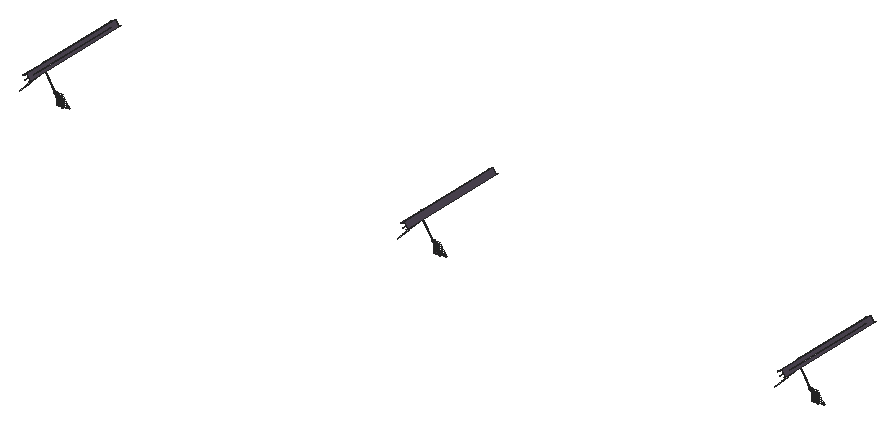
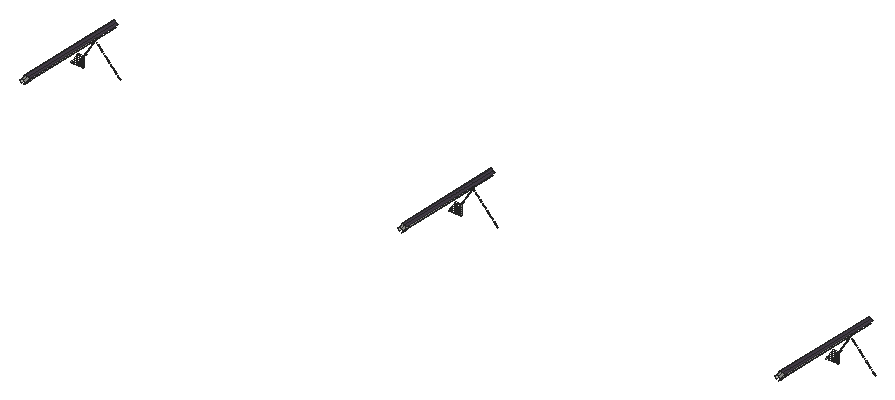
# SketchUp Ruby script. Lengths in inches.
U = 1.inch
M = Sketchup.active_model
def pt(a) = Geom::Point3d.new(a.map { |v| v * U })
def face(e, loops, mat)
  f = e.add_face(loops[0].map { |a| pt(a) })
  loops[1..].each { |l| e.add_face(l.map { |a| pt(a) }).erase! }
  f.material = f.back_material = mat if mat
  f
end
# faces: each face lists its corners as indices into pts; further lists are holes
def faces(e, pts, list, mat = nil) = list.each { |f| face(e, (f[0].is_a?(Array) ? f : [f]).map { |l| l.map { |i| pts[i] } }, mat) }
# xy, xz, yz: faces in a plane at the given z, y or x. An outline is a flat list of corners, or four numbers for a rectangle; further outlines are holes
def ring(l) = l.size == 4 ? [[l[0], l[1]], [l[2], l[1]], [l[2], l[3]], [l[0], l[3]]] : l.each_slice(2).to_a
def flat(e, list, mat, &to3) = list.each { |f| face(e, (f[0].is_a?(Array) ? f : [f]).map { |l| ring(l).map { |u, v| to3.(u, v) } }, mat) }
def xy(e, z, list, mat = nil) = flat(e, list, mat) { |x, y| [x, y, z] }
def xz(e, y, list, mat = nil) = flat(e, list, mat) { |x, z| [x, y, z] }
def yz(e, x, list, mat = nil) = flat(e, list, mat) { |y, z| [x, y, z] }
def lines(e, pts, list) = list.each { |a, b| e.add_line(pt(pts[a]), pt(pts[b])) }
# prism: a flat outline (further loops are holes) pulled along v
def prism(e, loops, v, mat = nil)
  f = face(e, loops, mat); d = Geom::Vector3d.new(v.map { |x| x * U })
  f.pushpull(f.normal.samedirection?(d) ? d.length : -d.length)
end
def box(e, o, s, mat = nil) = prism(e, [[o, [o[0] + s[0], o[1], o[2]], [o[0] + s[0], o[1] + s[1], o[2]], [o[0], o[1] + s[1], o[2]]]], [0, 0, s[2]], mat)
def at(x, y, z, deg = 0) = Geom::Transformation.translation(pt([x, y, z])) * Geom::Transformation.rotation(ORIGIN, Z_AXIS, deg.degrees)
def axes(o, x, y, z) = Geom::Transformation.new([*x, 0, *y, 0, *z, 0, *pt(o).to_a, 1])
def part(name) = M.definitions.add(name)
# library, detail: a bought-in or finely detailed component or shape, given as its bounding box
def library(name, o, s) = part(name).tap { |d| box(d.entities, o, s) }
def detail(e, o, s) = box(e.add_group.entities, o, s)
def put(e, d, t, mat = nil) = e.add_instance(d, t).tap { |i| i.material = mat if mat }
def group(e, t, mat = nil) = e.add_group.tap { |g| g.transformation = t; g.material = mat if mat }.entities
root = M.entities
M.materials.add("[Color M06]").color = [79, 71, 84]
xy(root,386.37,[[578.05,524.25,594.63,526.125],[1464.52,524.25,1481.09,526.125],[2350.98,524.25,2367.56,526.125]])
xy(root,387.5,[[578.05,524.25,593.91,526.125],[1464.52,524.25,1480.37,526.125],[2350.98,524.25,2366.84,526.125]])
xy(root,390.62,[[578.05,524.25,591.9,526.125],[1464.52,524.25,1478.37,526.125],[2350.98,524.25,2364.83,526.125]])
xy(root,391.75,[[578.05,524.25,591.18,526.125],[1464.52,524.25,1477.65,526.125],[2350.98,524.25,2364.11,526.125]])
xy(root,394.87,[[578.05,524.25,589.18,526.125],[1464.52,524.25,1475.64,526.125],[2350.98,524.25,2362.11,526.125]])
xy(root,396,[[578.05,524.25,588.46,526.125],[1464.52,524.25,1474.92,526.125],[2350.98,524.25,2361.39,526.125]])
xy(root,399.12,[[578.05,524.25,586.45,526.125],[1464.52,524.25,1472.92,526.125],[2350.98,524.25,2359.38,526.125]])
xy(root,400.25,[[578.05,524.25,585.73,526.125],[1464.52,524.25,1472.2,526.125],[2350.98,524.25,2358.66,526.125]])
xy(root,403.37,[[578.05,524.25,583.73,526.125],[1464.52,524.25,1470.19,526.125],[2350.98,524.25,2356.66,526.125]])
xy(root,404.5,[[578.05,524.25,583.01,526.125],[1464.52,524.25,1469.47,526.125],[2350.98,524.25,2355.9375,526.125]])
xy(root,407.62,[[578.05,524.25,581,526.125],[1464.52,524.25,1467.47,526.125],[2350.98,524.25,2353.93,526.125]])
xy(root,412.22,[[576.3,519.6875,578.05,521.5625],[1462.77,519.6875,1464.52,521.5625],[2349.23,519.6875,2350.98,521.5625],[576.3,521.5625,578.05,526.125],[1462.77,521.5625,1464.52,526.125],
  [2349.23,521.5625,2350.98,526.125]])
xz(root,521.5625,[[594.22,386.19,592.58,388.75,592.95,388.98,594.59,386.43],[1480.6875,386.19,1479.05,388.75,1479.42,388.98,1481.05,386.43],[2367.15,386.19,2365.51,388.75,2365.88,388.98,2367.52,386.43],[494.94,387.25,497.36,389.82,496.9,390.25,494.48,387.68],[1381.4,387.25,1383.82,389.82,1383.37,390.25,1380.94,387.68],
  [2267.86,387.25,2270.28,389.82,2269.83,390.25,2267.41,387.68],[592.03,389.61,590.39,392.17,590.76,392.4,592.4,389.85],[1478.49,389.61,1476.86,392.17,1477.22,392.4,1478.86,389.85],[2364.96,389.61,2363.32,392.17,2363.6875,392.4,2365.33,389.85],[498.23,390.75,500.66,393.33,500.2,393.75,497.78,391.18],
  [1384.7,390.75,1387.12,393.33,1386.66,393.75,1384.24,391.18],[2271.16,390.75,2273.58,393.33,2273.13,393.75,2270.71,391.18],[589.84,393.03,588.2,395.59,588.57,395.82,590.21,393.27],[1476.3,393.03,1474.66,395.59,1475.03,395.82,1476.67,393.27],[2362.77,393.03,2361.13,395.59,2361.5,395.82,2363.13,393.27],
  [501.53,394.26,503.95,396.83,503.5,397.26,501.08,394.6875],[1388,394.26,1390.42,396.83,1389.96,397.26,1387.54,394.6875],[2274.46,394.26,2276.88,396.83,2276.43,397.26,2274.01,394.6875],[587.64,396.45,586.01,399.01,586.375,399.24,588.01,396.69],[1474.11,396.45,1472.47,399.01,1472.84,399.24,1474.48,396.69],
  [2360.57,396.45,2358.94,399.01,2359.3,399.24,2360.94,396.69],[504.83,397.76,507.25,400.34,506.8,400.76,504.375,398.19],[1391.3,397.76,1393.72,400.34,1393.26,400.76,1390.84,398.19],[2277.76,397.76,2280.18,400.34,2279.73,400.76,2277.3,398.19],[585.45,399.875,583.81,402.43,584.18,402.66,585.82,400.11],
  [1471.92,399.875,1470.28,402.43,1470.65,402.66,1472.28,400.11],[2358.38,399.875,2356.74,402.43,2357.11,402.66,2358.75,400.11],[508.13,401.27,510.55,403.84,510.1,404.27,507.67,401.7],[1394.59,401.27,1397.01,403.84,1396.56,404.27,1394.14,401.7],[2281.06,401.27,2283.48,403.84,2283.02,404.27,2280.6,401.7],
  [583.26,403.29,581.62,405.85,581.99,406.08,583.63,403.53],[1469.72,403.29,1468.09,405.85,1468.45,406.08,1470.09,403.53],[2356.1875,403.29,2354.55,405.85,2354.92,406.08,2356.56,403.53],[511.43,404.77,513.85,407.34,513.39,407.77,510.97,405.2],[1397.89,404.77,1400.3125,407.34,1399.86,407.77,1397.4375,405.2],
  [2284.36,404.77,2286.78,407.34,2286.32,407.77,2283.9,405.2],[581.07,406.71,579.43,409.27,579.8,409.5,581.44,406.95],[1467.53,406.71,1465.89,409.27,1466.26,409.5,1467.9,406.95],[2354,406.71,2352.36,409.27,2352.73,409.5,2354.36,406.95],[514.73,408.28,517.15,410.85,516.69,411.28,514.27,408.7],
  [1401.19,408.28,1403.61,410.85,1403.16,411.28,1400.74,408.7],[2287.65,408.28,2290.08,410.85,2289.62,411.28,2287.2,408.7],[578.875,410.13,577.6875,411.99,578.05,412.22,579.24,410.37],[1465.34,410.13,1464.15,411.99,1464.52,412.22,1465.71,410.37],[2351.8,410.13,2350.61,411.99,2350.98,412.22,2352.17,410.37],
  [518.03,411.78,520.45,414.35,519.99,414.78,517.57,412.21],[1404.49,411.78,1406.91,414.35,1406.46,414.78,1404.03,412.21],[2290.95,411.78,2293.375,414.35,2292.92,414.78,2290.5,412.21],[577.6875,411.99,577.54,412.22,578.05,412.22],[1464.15,411.99,1464,412.22,1464.52,412.22],
  [2350.61,411.99,2350.46,412.22,2350.98,412.22],[577.54,412.22,578.05,412.22,577.61,412.92,577.24,412.6875],[1464,412.22,1464.52,412.22,1464.07,412.92,1463.7,412.6875],[2350.46,412.22,2350.98,412.22,2350.53,412.92,2350.16,412.6875],[576.68,413.55,577.05,413.79,575.86,415.64,575.49,415.41],
  [1463.15,413.55,1463.51,413.79,1462.33,415.64,1461.96,415.41],[2349.61,413.55,2349.98,413.79,2348.79,415.64,2348.42,415.41],[521.32,415.28,523.74,417.86,523.29,418.28,520.87,415.71],[1407.79,415.28,1410.21,417.86,1409.75,418.28,1407.33,415.71],[2294.25,415.28,2296.67,417.86,2296.22,418.28,2293.8,415.71],
  [575.49,415.41,575.86,415.64,575.41,416.34,575.04,416.11],[1461.96,415.41,1462.33,415.64,1461.875,416.34,1461.51,416.11],[2348.42,415.41,2348.79,415.64,2348.34,416.34,2347.97,416.11],[574.49,416.97,574.86,417.21,573.67,419.0625,573.3,418.83],[1460.95,416.97,1461.32,417.21,1460.13,419.0625,1459.77,418.83],
  [2347.42,416.97,2347.79,417.21,2346.6,419.0625,2346.23,418.83],[524.62,418.79,527.04,421.36,526.59,421.79,524.17,419.22],[1411.09,418.79,1413.51,421.36,1413.05,421.79,1410.63,419.22],[2297.55,418.79,2299.97,421.36,2299.52,421.79,2297.1,419.22],[573.3,418.83,573.67,419.0625,573.22,419.76,572.85,419.53],
  [1459.77,418.83,1460.13,419.0625,1459.68,419.76,1459.32,419.53],[2346.23,418.83,2346.6,419.0625,2346.15,419.76,2345.78,419.53],[572.3,420.39,572.66,420.63,571.48,422.48,571.11,422.25],[1458.76,420.39,1459.13,420.63,1457.94,422.48,1457.57,422.25],[2345.22,420.39,2345.59,420.63,2344.41,422.48,2344.04,422.25],
  [571.11,422.25,571.48,422.48,571.03,423.18,570.66,422.95],[1457.57,422.25,1457.94,422.48,1457.49,423.18,1457.12,422.95],[2344.04,422.25,2344.41,422.48,2343.96,423.18,2343.59,422.95],[527.92,422.29,530.34,424.86,529.89,425.29,527.47,422.72],[1414.38,422.29,1416.81,424.86,1416.35,425.29,1413.93,422.72],
  [2300.85,422.29,2303.27,424.86,2302.81,425.29,2300.39,422.72],[570.1,423.8125,570.47,424.05,569.28,425.9,568.92,425.67],[1456.57,423.8125,1456.9375,424.05,1455.75,425.9,1455.38,425.67],[2343.03,423.8125,2343.4,424.05,2342.21,425.9,2341.84,425.67],[568.92,425.67,569.28,425.9,568.83,426.6,568.47,426.37],
  [1455.38,425.67,1455.75,425.9,1455.3,426.6,1454.93,426.37],[2341.84,425.67,2342.21,425.9,2341.76,426.6,2341.39,426.37],[531.22,425.8,533.64,428.37,533.19,428.8,530.76,426.23],[1417.68,425.8,1420.1,428.37,1419.65,428.8,1417.23,426.23],[2304.15,425.8,2306.57,428.37,2306.11,428.8,2303.69,426.23],
  [567.91,427.23,568.28,427.47,567.09,429.32,566.72,429.09],[1454.375,427.23,1454.74,427.47,1453.56,429.32,1453.1875,429.09],[2340.84,427.23,2341.21,427.47,2340.02,429.32,2339.65,429.09],[566.72,429.09,567.09,429.32,566.64,430.02,566.27,429.79],[1453.1875,429.09,1453.56,429.32,1453.11,430.02,1452.74,429.79],
  [2339.65,429.09,2340.02,429.32,2339.57,430.02,2339.2,429.79],[534.52,429.3,536.9375,431.875,536.48,432.3,534.0625,429.73],[1420.98,429.3,1423.4,431.875,1422.95,432.3,1420.53,429.73],[2307.45,429.3,2309.87,431.875,2309.41,432.3,2306.99,429.73],[565.72,430.65,566.09,430.89,564.9,432.74,564.53,432.51],
  [1452.18,430.65,1452.55,430.89,1451.36,432.74,1451,432.51],[2338.65,430.65,2339.02,430.89,2337.83,432.74,2337.46,432.51],[564.53,432.51,564.9,432.74,564.45,433.44,564.08,433.21],[1451,432.51,1451.36,432.74,1450.91,433.44,1450.55,433.21],[2337.46,432.51,2337.83,432.74,2337.38,433.44,2337.01,433.21],
  [537.82,432.81,540.24,435.38,539.78,435.81,537.36,433.23],[1424.28,432.81,1426.7,435.38,1426.25,435.81,1423.83,433.23],[2310.74,432.81,2313.17,435.38,2312.71,435.81,2310.29,433.23],[563.53,434.07,563.89,434.31,562.71,436.16,562.34,435.93],[1449.99,434.07,1450.36,434.31,1449.17,436.16,1448.8,435.93],
  [2336.45,434.07,2336.82,434.31,2335.63,436.16,2335.27,435.93],[562.34,435.93,562.71,436.16,562.26,436.86,561.89,436.63],[1448.8,435.93,1449.17,436.16,1448.72,436.86,1448.35,436.63],[2335.27,435.93,2335.63,436.16,2335.18,436.86,2334.82,436.63],[541.12,436.31,543.54,438.88,543.08,439.31,540.66,436.74],
  [1427.58,436.31,1430,438.88,1429.55,439.31,1427.125,436.74],[2314.04,436.31,2316.46,438.88,2316.01,439.31,2313.59,436.74],[561.33,437.49,561.7,437.73,560.51,439.58,560.15,439.35],[1447.8,437.49,1448.17,437.73,1446.98,439.58,1446.61,439.35],[2334.26,437.49,2334.63,437.73,2333.44,439.58,2333.07,439.35],
  [560.15,439.35,560.51,439.58,560.0625,440.28,559.7,440.05],[1446.61,439.35,1446.98,439.58,1446.53,440.28,1446.16,440.05],[2333.07,439.35,2333.44,439.58,2332.99,440.28,2332.625,440.05],[544.41,439.8125,546.83,442.39,546.38,442.8125,543.96,440.24],[1430.88,439.8125,1433.3,442.39,1432.84,442.8125,1430.42,440.24],
  [2317.34,439.8125,2319.76,442.39,2319.31,442.8125,2316.89,440.24],[559.14,440.91,559.51,441.15,558.32,443,557.95,442.77],[1445.61,440.91,1445.97,441.15,1444.79,443,1444.42,442.77],[2332.07,440.91,2332.4375,441.15,2331.25,443,2330.88,442.77],[557.95,442.77,558.32,443,557.87,443.7,557.5,443.47],
  [1444.42,442.77,1444.79,443,1444.34,443.7,1443.97,443.47],[2330.88,442.77,2331.25,443,2330.8,443.7,2330.43,443.47],[547.71,443.32,550.13,445.89,549.68,446.32,547.26,443.75],[1434.18,443.32,1436.6,445.89,1436.14,446.32,1433.72,443.75],[2320.64,443.32,2323.0625,445.89,2322.61,446.32,2320.19,443.75],
  [556.95,444.33,557.32,444.57,556.13,446.42,555.76,446.1875],[1443.41,444.33,1443.78,444.57,1442.59,446.42,1442.22,446.1875],[2329.875,444.33,2330.24,444.57,2329.06,446.42,2328.6875,446.1875],[555.76,446.1875,556.13,446.42,555.68,447.125,555.3125,446.89],[1442.22,446.1875,1442.59,446.42,1442.14,447.125,1441.77,446.89],
  [2328.6875,446.1875,2329.06,446.42,2328.61,447.125,2328.24,446.89],[551.01,446.82,553.43,449.39,552.98,449.82,550.56,447.25],[1437.47,446.82,1439.9,449.39,1439.44,449.82,1437.02,447.25],[2323.9375,446.82,2326.36,449.39,2325.9,449.82,2323.48,447.25],[554.76,447.75,555.125,447.99,553.9375,449.84,553.57,449.61],
  [1441.22,447.75,1441.59,447.99,1440.4,449.84,1440.03,449.61],[2327.68,447.75,2328.05,447.99,2326.86,449.84,2326.5,449.61],[553.57,449.61,553.9375,449.84,553.56,450.4375,553.25,450.11],[1440.03,449.61,1440.4,449.84,1440.02,450.4375,1439.71,450.11],[2326.5,449.61,2326.86,449.84,2326.48,450.4375,2326.17,450.11],
  [553.25,450.11,553.1875,450.2,553.56,450.4375],[1439.71,450.11,1439.65,450.2,1440.02,450.4375],[2326.17,450.11,2326.11,450.2,2326.48,450.4375]])
xz(root,524.25,[[578.05,387.5,593.91,387.5,591.9,390.62,578.05,390.62],[1464.52,387.5,1480.37,387.5,1478.37,390.62,1464.52,390.62],[2350.98,387.5,2366.84,387.5,2364.83,390.62,2350.98,390.62],[578.05,391.75,591.18,391.75,589.18,394.87,578.05,394.87],[1464.52,391.75,1477.65,391.75,1475.64,394.87,1464.52,394.87],
  [2350.98,391.75,2364.11,391.75,2362.11,394.87,2350.98,394.87],[578.05,396,588.46,396,586.45,399.12,578.05,399.12],[1464.52,396,1474.92,396,1472.92,399.12,1464.52,399.12],[2350.98,396,2361.39,396,2359.38,399.12,2350.98,399.12],[578.05,400.25,585.73,400.25,583.73,403.37,578.05,403.37],
  [1464.52,400.25,1472.2,400.25,1470.19,403.37,1464.52,403.37],[2350.98,400.25,2358.66,400.25,2356.66,403.37,2350.98,403.37],[578.05,404.5,583.01,404.5,581,407.62,578.05,407.62],[1464.52,404.5,1469.47,404.5,1467.47,407.62,1464.52,407.62],[2350.98,404.5,2355.9375,404.5,2353.93,407.62,2350.98,407.62]],"[Color M06]")
xz(root,526.125,[[578.05,386.37,594.63,386.37,593.91,387.5,578.05,387.5],[1464.52,386.37,1481.09,386.37,1480.37,387.5,1464.52,387.5],[2350.98,386.37,2367.56,386.37,2366.84,387.5,2350.98,387.5],[604.81,387.5,607.53,387.5,605.53,390.62,602.8,390.62],[1491.27,387.5,1494,387.5,1491.99,390.62,1489.27,390.62],
  [2377.73,387.5,2380.46,387.5,2378.45,390.62,2375.73,390.62],[578.05,390.62,591.9,390.62,591.18,391.75,578.05,391.75],[1464.52,390.62,1478.37,390.62,1477.65,391.75,1464.52,391.75],[2350.98,390.62,2364.83,390.62,2364.11,391.75,2350.98,391.75],[578.05,394.87,589.18,394.87,588.46,396,578.05,396],
  [1464.52,394.87,1475.64,394.87,1474.92,396,1464.52,396],[2350.98,394.87,2362.11,394.87,2361.39,396,2350.98,396],[578.05,399.12,586.45,399.12,585.73,400.25,578.05,400.25],[1464.52,399.12,1472.92,399.12,1472.2,400.25,1464.52,400.25],[2350.98,399.12,2359.38,399.12,2358.66,400.25,2350.98,400.25],
  [578.05,403.37,583.73,403.37,583.01,404.5,578.05,404.5],[1464.52,403.37,1470.19,403.37,1469.47,404.5,1464.52,404.5],[2350.98,403.37,2356.66,403.37,2355.9375,404.5,2350.98,404.5],[578.05,407.62,581,407.62,580.125,409,578.05,409],[1464.52,407.62,1467.47,407.62,1466.59,409,1464.52,409],
  [2350.98,407.62,2353.93,407.62,2353.05,409,2350.98,409],[578.05,412.12,578.12,412.12,578.05,412.22],[1464.52,412.12,1464.58,412.12,1464.52,412.22],[2350.98,412.12,2351.05,412.12,2350.98,412.22]])
xz(root,526.125,[[578.05,409,580.125,409,578.12,412.12,578.05,412.12],[1464.52,409,1466.59,409,1464.58,412.12,1464.52,412.12],[2350.98,409,2353.05,409,2351.05,412.12,2350.98,412.12]],"[Color M06]")
xz(root,528.48,[[550.41,453.39,542.88,460.49,543.65,461.31,547.92,457.29],[550.41,453.39,547.92,457.29,551.1875,454.21],[1436.88,453.39,1429.34,460.49,1430.11,461.31,1434.38,457.29],[1436.88,453.39,1434.38,457.29,1437.65,454.21],[2323.34,453.39,2315.81,460.49,2316.58,461.31,2320.84,457.29],
  [2323.34,453.39,2320.84,457.29,2324.11,454.21],[551.1875,454.21,547.92,457.29,549.24,458.7,552.51,455.625],[1437.65,454.21,1434.38,457.29,1435.71,458.7,1438.98,455.625],[2324.11,454.21,2320.84,457.29,2322.17,458.7,2325.44,455.625],[547.92,457.29,543.65,461.31,544.98,462.72,549.24,458.7],
  [1434.38,457.29,1430.11,461.31,1431.44,462.72,1435.71,458.7],[2320.84,457.29,2316.58,461.31,2317.9,462.72,2322.17,458.7]])
xz(root,719.59,[[550.36,453.34,550.41,453.39,550.35,453.35],[1436.82,453.34,1436.88,453.39,1436.8125,453.35],[2323.29,453.34,2323.34,453.39,2323.28,453.35]])
xz(root,726.125,[[552.61,449.83,550.36,453.34,550.41,453.39,553.56,450.4375],[1439.07,449.83,1436.82,453.34,1436.88,453.39,1440.02,450.4375],[2325.54,449.83,2323.29,453.34,2323.34,453.39,2326.48,450.4375],[553.56,450.4375,550.41,453.39,545,461.85,549.93,465.01,557.61,453.03],[1440.02,450.4375,1436.88,453.39,1431.46,461.85,1436.39,465.01,1444.07,453.03],
  [2326.48,450.4375,2323.34,453.39,2317.92,461.85,2322.86,465.01,2330.53,453.03],[557.61,453.03,549.93,465.01,555.19,468.38,562.87,456.41],[1444.07,453.03,1436.39,465.01,1441.66,468.38,1449.33,456.41],[2330.53,453.03,2322.86,465.01,2328.12,468.38,2335.8,456.41],[550.36,453.34,550.35,453.35,550.41,453.39],
  [1436.82,453.34,1436.8125,453.35,1436.88,453.39],[2323.29,453.34,2323.28,453.35,2323.34,453.39]])
yz(root,578.05,[[524.25,387.5,526.125,390.62],[524.25,391.75,526.125,394.87],[524.25,396,526.125,399.12],[524.25,400.25,526.125,403.37],[524.25,404.5,526.125,407.62]])
yz(root,1464.52,[[524.25,387.5,526.125,390.62],[524.25,391.75,526.125,394.87],[524.25,396,526.125,399.12],[524.25,400.25,526.125,403.37],[524.25,404.5,526.125,407.62]])
yz(root,2350.98,[[524.25,387.5,526.125,390.62],[524.25,391.75,526.125,394.87],[524.25,396,526.125,399.12],[524.25,400.25,526.125,403.37],[524.25,404.5,526.125,407.62]])
p = [[590.76,519.6875,392.4],[590.76,521.5625,392.4],[590.39,521.5625,392.17],[590.39,519.6875,392.17],[2363.6875,519.6875,392.4],[2363.6875,521.5625,392.4],
  [2363.32,521.5625,392.17],[2363.32,519.6875,392.17],[588.57,519.6875,395.82],[588.57,521.5625,395.82],[588.2,521.5625,395.59],[588.2,519.6875,395.59],
  [2361.5,519.6875,395.82],[2361.5,521.5625,395.82],[2361.13,521.5625,395.59],[2361.13,519.6875,395.59],[586.375,519.6875,399.24],[586.375,521.5625,399.24],
  [586.01,521.5625,399.01],[586.01,519.6875,399.01],[2359.3,519.6875,399.24],[2359.3,521.5625,399.24],[2358.94,521.5625,399.01],[2358.94,519.6875,399.01],
  [584.18,519.6875,402.66],[584.18,521.5625,402.66],[583.81,521.5625,402.43],[583.81,519.6875,402.43],[2357.11,519.6875,402.66],[2357.11,521.5625,402.66],
  [2356.74,521.5625,402.43],[2356.74,519.6875,402.43],[581.99,519.6875,406.08],[581.99,521.5625,406.08],[581.62,521.5625,405.85],[581.62,519.6875,405.85],
  [2354.92,519.6875,406.08],[2354.92,521.5625,406.08],[2354.55,521.5625,405.85],[2354.55,519.6875,405.85],[579.8,519.6875,409.5],[579.8,521.5625,409.5],
  [579.43,521.5625,409.27],[579.43,519.6875,409.27],[2352.73,519.6875,409.5],[2352.73,521.5625,409.5],[2352.36,521.5625,409.27],[2352.36,519.6875,409.27],
  [553.56,528.48,450.4375],[553.56,719.59,450.4375],[553.56,726.125,450.4375],[553.56,731.75,450.4375],[550.41,731.75,453.39],[550.41,726.125,453.39],
  [550.41,719.59,453.39],[550.41,528.48,453.39],[1440.02,528.48,450.4375],[1440.02,719.59,450.4375],[1440.02,726.125,450.4375],[1440.02,731.75,450.4375],
  [1436.88,731.75,453.39],[1436.88,726.125,453.39],[1436.88,719.59,453.39],[1436.88,528.48,453.39],[2326.48,528.48,450.4375],[2326.48,719.59,450.4375],
  [2326.48,726.125,450.4375],[2326.48,731.75,450.4375],[2323.34,731.75,453.39],[2323.34,726.125,453.39],[2323.34,719.59,453.39],[2323.34,528.48,453.39],
  [557.61,726.125,453.03],[562.87,726.125,456.41],[562.87,732.2,456.41],[557.61,732.2,453.03],[1444.07,726.125,453.03],[1449.33,726.125,456.41],
  [1449.33,732.2,456.41],[1444.07,732.2,453.03],[2330.53,726.125,453.03],[2335.8,726.125,456.41],[2335.8,732.2,456.41],[2330.53,732.2,453.03],
  [550.36,719.59,453.34],[550.36,467.1875,453.34],[550.41,467.1875,453.39],[1436.82,719.59,453.34],[1436.82,467.1875,453.34],[1436.88,467.1875,453.39],
  [2323.29,719.59,453.34],[2323.29,467.1875,453.34],[2323.34,467.1875,453.39],[542.88,528.48,460.49],[542.88,731.75,460.49],[547.92,528.48,457.29],
  [545,528.48,461.85],[545,719.59,461.85],[1429.34,528.48,460.49],[1429.34,731.75,460.49],[1434.38,528.48,457.29],[1431.46,528.48,461.85],
  [1431.46,719.59,461.85],[2315.81,528.48,460.49],[2315.81,731.75,460.49],[2320.84,528.48,457.29],[2317.92,528.48,461.85],[2317.92,719.59,461.85],
  [545,726.125,461.85],[550.35,719.59,453.35],[550.35,726.125,453.35],[1431.46,726.125,461.85],[1436.8125,719.59,453.35],[1436.8125,726.125,453.35],
  [2317.92,726.125,461.85],[2323.28,719.59,453.35],[2323.28,726.125,453.35],[562.87,467.1875,456.41],[555.19,726.125,468.38],[555.19,467.1875,468.38],
  [1449.33,467.1875,456.41],[1441.66,726.125,468.38],[1441.66,467.1875,468.38],[2335.8,467.1875,456.41],[2328.12,726.125,468.38],[2328.12,467.1875,468.38],
  [549.93,726.125,465.01],[545,467.1875,461.85],[545.54,467.1875,462.19],[549.93,467.1875,465.01],[1436.39,726.125,465.01],[1431.46,467.1875,461.85],
  [1432,467.1875,462.19],[1436.39,467.1875,465.01],[2322.86,726.125,465.01],[2317.92,467.1875,461.85],[2318.46,467.1875,462.19],[2322.86,467.1875,465.01],
  [1444.07,467.1875,453.03],[1439.07,719.59,449.83],[1439.07,726.125,449.83],[1486.54,526.125,386.37],[1489.27,526.125,386.37],[1483.82,526.125,386.37],
  [1481.09,526.125,386.37],[1481.09,526.125,390.62],[1483.82,526.125,390.62],[1483.1,526.125,387.5],[1480.37,526.125,387.5],[1485.82,526.125,387.5],
  [1486.54,526.125,390.62],[1489.27,526.125,390.62],[1491.27,526.125,387.5],[1488.55,526.125,387.5],[1478.37,526.125,390.62],[1489.27,526.125,394.87],
  [1491.27,526.125,391.75],[1478.37,526.125,394.87],[1481.09,526.125,394.87],[1480.37,526.125,391.75],[1477.65,526.125,391.75],[1483.1,526.125,391.75],
  [1486.54,526.125,394.87],[1488.55,526.125,391.75],[1485.82,526.125,391.75],[1483.82,526.125,394.87],[1475.64,526.125,394.87],[1475.64,526.125,399.12],
  [1478.37,526.125,399.12],[1477.65,526.125,396],[1474.92,526.125,396],[1481.09,526.125,399.12],[1483.82,526.125,399.12],[1485.82,526.125,396],
  [1483.1,526.125,396],[1488.55,526.125,396],[1480.37,526.125,396],[1486.54,526.125,399.12],[1472.92,526.125,399.12],[1478.37,526.125,403.37],
  [1481.09,526.125,403.37],[1480.37,526.125,400.25],[1477.65,526.125,400.25],[1474.92,526.125,400.25],[1483.82,526.125,403.37],[1485.82,526.125,400.25],
  [1483.1,526.125,400.25],[1475.64,526.125,403.37],[1472.92,526.125,403.37],[1472.2,526.125,400.25],[1470.19,526.125,403.37],[1472.92,526.125,407.62],
  [1475.64,526.125,407.62],[1477.65,526.125,404.5],[1474.92,526.125,404.5],[1478.37,526.125,407.62],[1481.09,526.125,407.62],[1472.2,526.125,404.5],
  [1480.37,526.125,404.5],[1483.1,526.125,404.5],[1470.19,526.125,407.62],[1469.47,526.125,404.5],[1467.47,526.125,407.62],[1470.19,526.125,412.12],
  [1472.92,526.125,412.12],[1474.92,526.125,409],[1472.2,526.125,409],[1475.64,526.125,412.12],[1480.37,526.125,409],[1477.65,526.125,409],
  [1469.47,526.125,409],[1478.37,526.125,412.12],[1467.47,526.125,412.12],[1466.59,526.125,409],[1464.58,526.125,412.12],[2367.56,526.125,386.37],
  [2370.28,526.125,386.37],[2364.83,526.125,390.62],[2367.56,526.125,390.62],[2373.01,526.125,386.37],[2375.73,526.125,386.37],[2356.66,526.125,407.62],
  [2359.38,526.125,407.62],[2361.39,526.125,404.5],[2358.66,526.125,404.5],[2369.5625,526.125,404.5],[2366.84,526.125,404.5],[2362.11,526.125,407.62],
  [2364.11,526.125,404.5],[2355.9375,526.125,404.5],[2364.83,526.125,407.62],[2367.56,526.125,407.62],[2364.83,526.125,399.12],[2367.56,526.125,399.12],
  [2375.01,526.125,396],[2372.29,526.125,396],[2366.84,526.125,396],[2364.11,526.125,396],[2361.39,526.125,396],[2370.28,526.125,399.12],
  [2369.5625,526.125,396],[2362.11,526.125,399.12],[2373.01,526.125,399.12],[2362.11,526.125,394.87],[2364.83,526.125,394.87],[2356.66,526.125,412.12],
  [2359.38,526.125,412.12],[2361.39,526.125,409],[2358.66,526.125,409],[2362.11,526.125,412.12],[2364.83,526.125,412.12],[2355.9375,526.125,409],
  [2351.05,526.125,412.12],[2353.93,526.125,412.12],[2364.11,526.125,409],[2366.84,526.125,409],[2353.05,526.125,409],[2359.38,526.125,403.37],
  [2362.11,526.125,403.37],[2369.5625,526.125,387.5],[2366.84,526.125,387.5],[2373.01,526.125,390.62],[2375.73,526.125,390.62],[2375.01,526.125,387.5],
  [2372.29,526.125,387.5],[2367.56,526.125,403.37],[2370.28,526.125,403.37],[2377.73,526.125,387.5],[2364.11,526.125,400.25],[2361.39,526.125,400.25],
  [2364.83,526.125,403.37],[2372.29,526.125,400.25],[2369.5625,526.125,400.25],[2358.66,526.125,400.25],[2366.84,526.125,400.25],[2370.28,526.125,390.62],
  [2373.01,526.125,394.87],[2375.73,526.125,394.87],[2367.56,526.125,394.87],[2377.73,526.125,391.75],[2375.01,526.125,391.75],[2359.38,526.125,399.12],
  [2370.28,526.125,394.87],[2372.29,526.125,391.75],[2369.5625,526.125,391.75],[2366.84,526.125,391.75],[2364.11,526.125,391.75],[2353.93,526.125,407.62],
  [2356.66,526.125,403.37],[2330.53,467.1875,453.03],[2325.54,719.59,449.83],[2325.54,726.125,449.83],[591.9,526.125,394.87],[594.63,526.125,394.87],
  [586.45,526.125,399.12],[589.18,526.125,399.12],[594.63,526.125,390.62],[597.35,526.125,390.62],[597.35,526.125,394.87],[596.63,526.125,400.25],
  [593.91,526.125,400.25],[604.81,526.125,391.75],[602.08,526.125,391.75],[591.18,526.125,400.25],[600.08,526.125,390.62],[602.8,526.125,394.87],
  [600.08,526.125,394.87],[599.36,526.125,391.75],[581,526.125,407.62],[583.73,526.125,407.62],[596.63,526.125,391.75],[583.73,526.125,403.37],
  [586.45,526.125,403.37],[593.91,526.125,391.75],[591.18,526.125,391.75],[557.61,467.1875,453.03],[552.61,719.59,449.83],[552.61,726.125,449.83],
  [599.36,526.125,396],[596.63,526.125,396],[597.35,526.125,399.12],[600.08,526.125,399.12],[589.18,526.125,394.87],[593.91,526.125,396],
  [591.18,526.125,396],[591.9,526.125,399.12],[588.46,526.125,396],[594.63,526.125,399.12],[583.73,526.125,412.12],[586.45,526.125,412.12],
  [589.18,526.125,412.12],[591.9,526.125,412.12],[591.18,526.125,409],[588.46,526.125,409],[596.63,526.125,387.5],[593.91,526.125,387.5],
  [589.18,526.125,403.37],[581,526.125,412.12],[594.63,526.125,403.37],[597.35,526.125,403.37],[599.36,526.125,387.5],[588.46,526.125,400.25],
  [591.9,526.125,403.37],[599.36,526.125,400.25],[583.01,526.125,409],[580.125,526.125,409],[578.12,526.125,412.12],[585.73,526.125,400.25],
  [593.91,526.125,409],[585.73,526.125,409],[602.8,526.125,390.62],[602.08,526.125,387.5],[604.81,526.125,387.5],[594.63,526.125,386.37],
  [597.35,526.125,386.37],[591.9,526.125,390.62],[586.45,526.125,407.62],[589.18,526.125,407.62],[591.9,526.125,407.62],[594.63,526.125,407.62],
  [600.08,526.125,386.37],[602.8,526.125,386.37],[588.46,526.125,404.5],[585.73,526.125,404.5],[593.91,526.125,404.5],[591.18,526.125,404.5],
  [583.01,526.125,404.5],[596.63,526.125,404.5],[602.08,526.125,396]]
faces(root,p,[[0,1,2,3],[4,5,6,7],[8,9,10,11],[12,13,14,15],[16,17,18,19],[20,21,22,23],[24,25,26,27],[28,29,30,31],
  [32,33,34,35],[36,37,38,39],[40,41,42,43],[44,45,46,47],[48,49,50,51,52,53,54,55],[56,57,58,59,60,61,62,63],[64,65,66,67,68,69,70,71],[72,73,74,75],
  [76,77,78,79],[80,81,82,83],[54,84,85,86,55],[62,87,88,89,63],[70,90,91,92,71],[93,55,54,53,52,94],[54,55,95,96,97],[98,63,62,61,60,99],
  [62,63,100,101,102],[103,71,70,69,68,104],[70,71,105,106,107],[53,54,97,108],[109,54,53,110],[61,62,102,111],[112,62,61,113],[69,70,107,114],
  [115,70,69,116]])
faces(root,p,[[117,73,118,119],[120,77,121,122],[123,81,124,125],[126,108,97,96,127,128,129],[130,111,102,101,131,132,133],[134,114,107,106,135,136,137],[126,129,119,118],[130,133,122,121],
  [134,137,125,124]],"[Color M06]")
lines(root,p,[[138,76],[139,140],[141,142],[143,141],[144,143],[145,146],[147,148],[149,147],[150,151],[152,153],[153,149],[146,150],
  [154,145],[155,156],[157,158],[159,160],[161,159],[162,155],[163,164],[156,163],[164,161],[165,162],[158,165],[166,157],
  [167,168],[169,170],[168,171],[171,172],[173,174],[175,173],[176,169],[172,177],[174,176],[178,167],[179,180],[181,182],
  [182,183],[180,184],[185,186],[187,179],[186,181],[188,187],[183,189],[190,188],[191,192],[193,194],[195,196],[194,197],
  [192,195],[198,193],[199,198],[200,191],[197,201],[202,200],[203,204],[205,206],[204,207],[208,209],[206,210],[207,211],
  [209,205],[212,203],[210,213],[214,212],[215,216],[217,218],[219,220],[216,219],[221,222],[223,224],[225,226],[222,227],
  [226,228],[224,229],[230,231],[227,230],[228,223],[232,233],[234,235],[236,237],[237,238],[233,239],[235,240],[241,232],
  [240,236],[239,242],[243,244],[245,246],[247,248],[249,250],[246,249],[248,251],[252,253],[254,247],[255,254],[251,256],
  [253,245],[257,258],[259,260],[261,262],[263,264],[265,266],[267,263],[264,259],[268,269],[270,265],[271,272],[269,273],
  [258,270],[274,268],[275,261],[218,275],[272,274],[276,277],[244,278],[279,280],[281,241],[278,282],[277,279],[283,284],
  [280,283],[285,286],[282,276],[284,285],[287,221],[288,257],[289,80],[290,291],[292,293],[294,295],[296,297],[293,298],
  [299,300],[301,302],[300,303],[297,304],[305,301],[306,305],[302,307],[308,309],[307,310],[311,312],[313,314],[298,306],
  [310,313],[315,72],[316,317],[318,319],[320,321],[322,292],[323,324],[295,325],[324,326],[327,320],[319,323],[328,329],
  [330,331],[332,333],[334,335],[312,336],[337,328],[338,339],[329,330],[340,334],[303,341],[342,338],[343,299],[344,345],
  [346,337],[341,347],[348,332],[336,342],[349,344],[304,350],[333,349],[351,340],[352,351],[353,354],[355,296],[356,357],
  [358,359],[357,358],[309,356],[360,361],[362,363],[364,365],[363,366],[365,362],[354,360],[367,364],[325,327],[368,318]])
